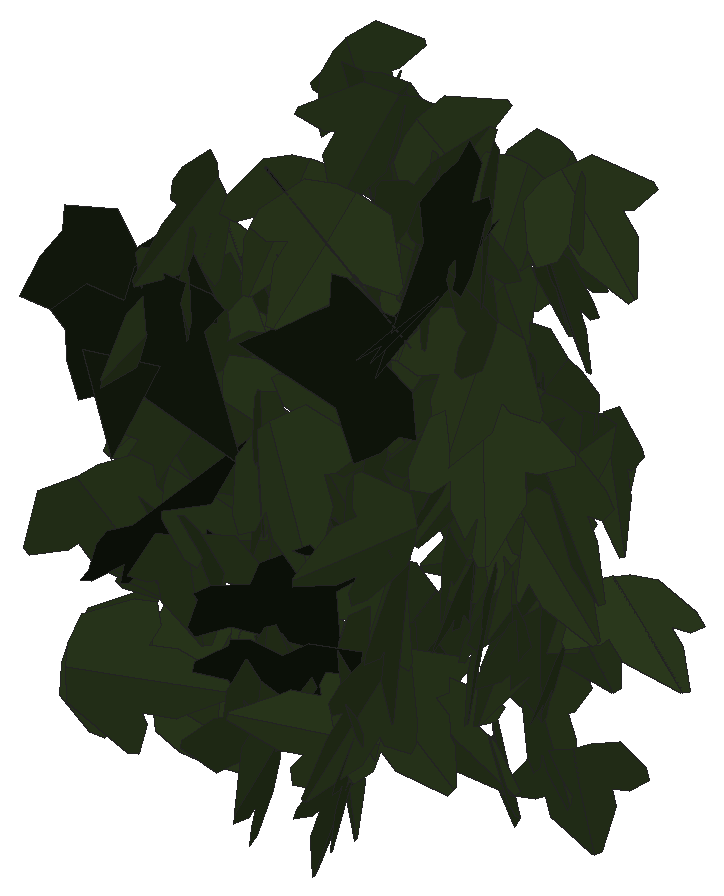
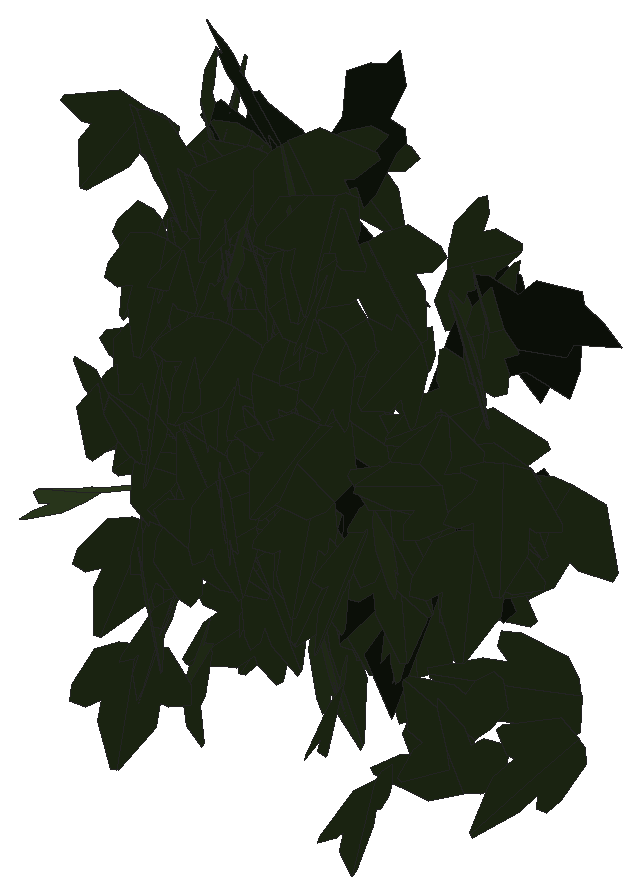
# SketchUp Ruby script. Lengths in inches.
U = 1.inch
M = Sketchup.active_model
def pt(a) = Geom::Point3d.new(a.map { |v| v * U })
def face(e, loops, mat)
  f = e.add_face(loops[0].map { |a| pt(a) })
  loops[1..].each { |l| e.add_face(l.map { |a| pt(a) }).erase! }
  f.material = f.back_material = mat if mat
  f
end
# faces: each face lists its corners as indices into pts; further lists are holes
def faces(e, pts, list, mat = nil) = list.each { |f| face(e, (f[0].is_a?(Array) ? f : [f]).map { |l| l.map { |i| pts[i] } }, mat) }
# xy, xz, yz: faces in a plane at the given z, y or x. An outline is a flat list of corners, or four numbers for a rectangle; further outlines are holes
def ring(l) = l.size == 4 ? [[l[0], l[1]], [l[2], l[1]], [l[2], l[3]], [l[0], l[3]]] : l.each_slice(2).to_a
def flat(e, list, mat, &to3) = list.each { |f| face(e, (f[0].is_a?(Array) ? f : [f]).map { |l| ring(l).map { |u, v| to3.(u, v) } }, mat) }
def xy(e, z, list, mat = nil) = flat(e, list, mat) { |x, y| [x, y, z] }
def xz(e, y, list, mat = nil) = flat(e, list, mat) { |x, z| [x, y, z] }
def yz(e, x, list, mat = nil) = flat(e, list, mat) { |y, z| [x, y, z] }
def lines(e, pts, list) = list.each { |a, b| e.add_line(pt(pts[a]), pt(pts[b])) }
# prism: a flat outline (further loops are holes) pulled along v
def prism(e, loops, v, mat = nil)
  f = face(e, loops, mat); d = Geom::Vector3d.new(v.map { |x| x * U })
  f.pushpull(f.normal.samedirection?(d) ? d.length : -d.length)
end
def box(e, o, s, mat = nil) = prism(e, [[o, [o[0] + s[0], o[1], o[2]], [o[0] + s[0], o[1] + s[1], o[2]], [o[0], o[1] + s[1], o[2]]]], [0, 0, s[2]], mat)
def at(x, y, z, deg = 0) = Geom::Transformation.translation(pt([x, y, z])) * Geom::Transformation.rotation(ORIGIN, Z_AXIS, deg.degrees)
def axes(o, x, y, z) = Geom::Transformation.new([*x, 0, *y, 0, *z, 0, *pt(o).to_a, 1])
def part(name) = M.definitions.add(name)
# library, detail: a bought-in or finely detailed component or shape, given as its bounding box
def library(name, o, s) = part(name).tap { |d| box(d.entities, o, s) }
def detail(e, o, s) = box(e.add_group.entities, o, s)
def put(e, d, t, mat = nil) = e.add_instance(d, t).tap { |i| i.material = mat if mat }
def group(e, t, mat = nil) = e.add_group.tap { |g| g.transformation = t; g.material = mat if mat }.entities
root = M.entities
M.materials.add("efeu1").color = [18, 25, 13]
M.materials.add("efeu2").color = [43, 57, 29]
c1 = part("ivyleaf_10")
p = [[0,0.5,-0.03],[-0.0625,2.02,-0.43],[-0.19,2.01,-0.46],[-0.54,1.05,-0.29],[-0.52,0.625,-0.18],[-0.83,0.76,-0.28],
  [-1.16,0.64,-0.33],[-1.15,0.33,-0.24],[-0.77,-0.39,0.02],[-0.3,-0.51,0.16],[0.04,-0.48,0.23],[-0.02,2.01,-0.4375],
  [-0.06,2.01,-0.43],[0.04,-0.49,0.23],[0.67,-0.49,0.14],[1.38,0.36,-0.2],[1.375,0.51,-0.24],[0.81,0.65,-0.19],
  [0.62,0.59,-0.15],[0.6,1.09,-0.28],[0.5,1.23,-0.31]]
faces(c1.entities,p,[[0,1,2,3,4,5,6,7,8,9,10],[11,12,0,13,14,15,16,17,18,19,20]],"efeu2")
c2 = part("ivyleaf_9")
p = [[1.54,2.16,1.25],[1.36,2.04,1.19],[-0.21,0.99,0.68],[-0.71,1.11,0.82],[-0.85,0.86,0.67],[-0.8,0.17,0.21],
  [-0.9,-0.01,0.1],[-0.67,-0.16,-0.02],[-0.08,-0.08,-0.05],[-0.03,-0.6,-0.4],[0.65,-0.88,-0.66],[0.83,-0.6,-0.49],
  [1.29,-0.42,-0.43],[1.8125,-0.07,-0.26],[1.21,0.44,0.15]]
faces(c2.entities,p,[[0,1,2,3,4,5,6,7,8,9,10,11,12,13,14]],"efeu1")
put(root,c1,axes([598.12,137.04,169.68],[-0.00094,-0.16747,0.7103],[0.19279,-0.68513,-0.16128],[0.70385,0.18744,0.04512]))
put(root,c2,axes([597.98,136.37,169.84],[-0.18069,-0.20058,-0.71209],[0.44721,0.55432,-0.26962],[0.58933,-0.48214,-0.01373]))
put(root,c2,axes([597.75,136.77,170.26],[-0.54152,-0.45185,-0.36971],[0.27813,0.24371,-0.70523],[0.51332,-0.60872,-0.00792]))
put(root,c1,axes([599.44,137.05,164.22],[-0.10246,0.01438,0.77216],[0.4757,-0.61244,0.07452],[0.60839,0.48129,0.07177]))
put(root,c1,axes([599.68,136.74,168.8],[-0.16104,0.54448,-0.30768],[0.07215,-0.29943,-0.56763],[-0.62123,-0.17592,0.01384]))
put(root,c1,axes([598.22,137.02,169.99],[0.02528,-0.04858,-0.68437],[0.3438,-0.59175,0.05471],[-0.59374,-0.34472,0.00254]))
put(root,c2,axes([600.16,136.57,171.97],[0.70624,-0.29216,-0.01882],[-0.01644,0.00948,-0.76428],[0.2923,0.70642,0.00247]))
put(root,c2,axes([601.4,136.67,170.17],[-0.23014,0.01953,-0.72477],[-0.64627,-0.35021,0.19577],[-0.32865,0.67499,0.12254]))
put(root,c1,axes([597.39,136.52,167.09],[-0.59466,-0.39368,-0.37778],[0.34415,0.16298,-0.71156],[0.42339,-0.6854,0.04779]))
put(root,c1,axes([600.03,136.57,168.53],[0.16273,0.7537,0.11512],[0.02463,0.11246,-0.77107],[-0.76204,0.16458,-0.00034]))
put(root,c1,axes([599.46,136.9,164.56],[-0.29472,-0.72736,-0.06906],[-0.02636,-0.06383,0.7848],[-0.73015,0.2959,-0.00046]))
put(root,c1,axes([600.63,137.0625,164.85],[0.08816,0.13501,0.65877],[-0.4395,-0.49131,0.1595],[0.50897,-0.44763,0.02363]))
put(root,c1,axes([601.49,136.92,167.0625],[0.31671,-0.70982,0.08083],[0.16055,-0.01543,-0.76463],[0.69613,0.3265,0.13958]))
put(root,c2,axes([597.81,136.625,166.375],[0.31189,0.68993,0.05468],[-0.04652,-0.03895,0.75669],[0.69052,-0.31425,0.02628]))
put(root,c1,axes([601.01,137.19,165.58],[0.02451,0.54049,-0.53466],[-0.26029,-0.49664,-0.51399],[-0.71431,0.19953,0.16895]))
put(root,c1,axes([600.49,137.04,171.55],[0.60036,0.27951,-0.31616],[-0.28387,-0.13931,-0.66221],[-0.31225,0.66407,-0.00585]))
put(root,c2,axes([602.32,137.12,172.32],[-0.67019,0.21596,-0.35153],[0.32806,-0.12767,-0.70388],[-0.25017,-0.74594,0.0187]))
put(root,c1,axes([600.92,137.42,167.41],[-0.02445,-0.02156,0.66723],[-0.01179,-0.66756,-0.022],[0.66747,-0.01258,0.02405]))
put(root,c1,axes([598.27,137.41,170.9],[0.0302,0.25247,-0.67775],[-0.11166,-0.66857,-0.25403],[-0.71457,0.11515,0.01106]))
put(root,c2,axes([600,136.68,165.81],[0.37753,0.58895,-0.35695],[-0.29716,-0.22791,-0.69033],[-0.62127,0.4669,0.11329]))
put(root,c1,axes([598.33,137.03,167.96],[-0.56505,-0.28517,0.36611],[-0.32868,-0.16131,-0.63292],[0.32761,-0.65368,-0.00353]))
put(root,c2,axes([602.11,136.92,171.36],[-0.46704,0.62886,-0.13687],[-0.02331,-0.18552,-0.77289],[-0.64316,-0.44993,0.12739]))
put(root,c2,axes([599.72,136.51,166.75],[0.45051,0.6646,0.04239],[0.02729,0.03271,-0.80289],[-0.66539,0.45132,-0.00423]))
put(root,c1,axes([598.26,137.07,166.2],[-0.51043,0.08714,-0.52601],[-0.52695,0.02846,0.51607],[0.08121,0.7324,0.04253]))
put(root,c1,axes([597.2,136.88,164.63],[-0.03493,-0.00707,-0.79493],[0.78918,0.09553,-0.03553],[0.09575,-0.78994,0.00281]))
put(root,c1,axes([598.38,137.01,166.47],[-0.57362,-0.34446,-0.03193],[0.02728,0.01659,-0.6691],[0.34486,-0.57427,-0.00018]))
put(root,c1,axes([602.31,137.39,170.84],[-0.33697,0.46787,0.50899],[0.30301,-0.409,0.57656],[0.62141,0.45314,-0.00513]))
put(root,c1,axes([600.5,137.27,164.4],[0.17307,-0.73707,0.09646],[-0.00535,-0.10027,-0.75661],[0.74334,0.17089,-0.02791]))
put(root,c1,axes([600.52,137.39,164.75],[0.39169,-0.63117,0.09926],[0.06472,-0.07664,-0.74269],[0.63564,0.39673,0.01446]))
put(root,c1,axes([601.74,137.69,167.62],[-0.04421,-0.28985,-0.63625],[0.32943,-0.57095,0.23721],[-0.61669,-0.28422,0.17233]))
put(root,c1,axes([599.38,137.31,165.3125],[-0.45285,0.32436,-0.36513],[0.30643,-0.19903,-0.55685],[-0.3803,-0.54661,-0.01391]))
put(root,c1,axes([600.68,137.07,165.8],[-0.26645,0.49635,0.38567],[-0.22343,0.31674,-0.562],[-0.58752,-0.34556,0.03883]))
put(root,c1,axes([602.18,137.51,170.26],[0.74901,0.04342,-0.11895],[-0.11994,0.01445,-0.74997],[-0.04061,0.75826,0.02111]))
put(root,c1,axes([598.02,137.64,170.22],[0.47169,-0.57647,-0.03784],[-0.02352,0.02965,-0.74486],[0.57723,0.47228,0.00057]))
put(root,c1,axes([598.53,137.59,168.26],[-0.19879,-0.0151,-0.63074],[0.61622,-0.14657,-0.1907],[-0.1354,-0.64488,0.05811]))
put(root,c1,axes([598.34,137.11,167.36],[-0.00658,0.49727,0.53231],[-0.02821,0.53176,-0.4971],[-0.7279,-0.0251,0.01446]))
put(root,c1,axes([602.18,137.5625,169.11],[0.53495,0.52861,0.02722],[0.01948,0.01902,-0.75206],[-0.52895,0.5353,-0.00016]))
put(root,c1,axes([601.92,137.9375,166.67],[0.36629,-0.32575,0.49459],[0.34918,-0.35092,-0.48973],[0.47834,0.50562,-0.02125]))
put(root,c1,axes([597.71,137.64,168.11],[0.55127,-0.0916,-0.40363],[-0.40034,0.05261,-0.55871],[0.10504,0.68121,-0.01112]))
put(root,c1,axes([600.5,137.71,166.33],[0.68399,-0.2207,-0.05303],[-0.04822,0.02324,-0.71868],[0.2218,0.68565,0.00729]))
put(root,c1,axes([599.8,137.98,168.31],[-0.23048,-0.28788,0.54307],[-0.32592,-0.4345,-0.36865],[0.52113,-0.39907,0.00963]))
put(root,c1,axes([598.37,137.21,168.58],[0.02744,-0.07316,0.66296],[-0.05757,0.66079,0.0753],[-0.6645,-0.06027,0.02086]))
put(root,c1,axes([601.9,138.05,172.12],[0.34235,-0.40903,0.4743],[0.37577,-0.29829,-0.52848],[0.50106,0.50317,0.07227]))
put(root,c1,axes([600.875,137.38,165.3],[0.28122,0.56152,0.42564],[0.10198,0.42103,-0.62281],[-0.69719,0.28808,0.08059]))
put(root,c1,axes([601.64,137.75,171.46],[-0.67701,0.08676,-0.08449],[0.08282,-0.01835,-0.6825],[-0.08835,-0.68201,0.00762]))
put(root,c1,axes([601.78,137.82,167.12],[0.16628,-0.57663,-0.35816],[-0.10484,0.3425,-0.60011],[0.67066,0.19651,-0.00501]))
put(root,c1,axes([601.08,137.99,166.36],[-0.50462,-0.05558,0.38763],[-0.38182,-0.07059,-0.50717],[0.08698,-0.63239,0.02255]))
put(root,c1,axes([601.42,137.63,171.13],[0.19483,-0.42232,-0.55143],[0.02762,0.57697,-0.43212],[0.69402,0.0956,0.172]))
put(root,c1,axes([600.51,137.72,167.77],[-0.33742,0.41011,0.36563],[-0.22972,0.28446,-0.53107],[-0.49911,-0.40818,-0.00275]))
put(root,c1,axes([600.75,138.24,165.62],[-0.0006,-0.65883,0.16871],[0.00446,-0.16871,-0.65881],[0.68007,0.00052,0.00447]))
put(root,c1,axes([599.04,138.13,170.99],[0.4283,0.49079,-0.25962],[-0.26584,-0.10659,-0.64007],[-0.48745,0.48937,0.12095]))
put(root,c1,axes([599.74,138.12,164.24],[-0.18973,0.57199,-0.22008],[0.08381,-0.20401,-0.60246],[-0.60711,-0.20692,-0.01439]))
put(root,c1,axes([598.625,138.09,169.68],[-0.49263,0.25831,-0.34202],[0.30586,-0.15315,-0.55622],[-0.30025,-0.57983,-0.00546]))
put(root,c1,axes([596.53,137.59,164.24],[0.07282,0.38468,0.60598],[0.09011,0.59937,-0.39131],[-0.71209,0.11518,0.01245]))
put(root,c1,axes([601.12,138.03,164.91],[-0.44738,-0.05685,-0.4497],[0.45027,0.01689,-0.45009],[0.0521,-0.63411,0.02833]))
put(root,c1,axes([597.9,137.94,163.63],[0.63713,0.3037,-0.20744],[0.18744,0.08888,0.70581],[0.31644,-0.66413,-0.00041]))
put(root,c1,axes([601.05,138.375,168.23],[-0.03152,-0.60197,0.25097],[-0.016,-0.25048,-0.60279],[0.652,-0.03524,-0.00266]))
put(root,c1,axes([597.26,138.45,167.41],[0.04502,0.48939,-0.48758],[-0.24893,-0.4443,-0.46893],[-0.64441,0.20582,0.14708]))
put(root,c1,axes([598.59,138.48,167.34],[0.24763,-0.54842,0.35009],[0.16405,-0.30985,-0.60144],[0.62961,0.29643,0.01901]))
put(root,c1,axes([598.75,138.14,166.65],[-0.63625,-0.16491,0.17004],[-0.16403,-0.04484,-0.65727],[0.17089,-0.65705,0.00218]))
put(root,c1,axes([602.01,138.29,168.97],[-0.02467,-0.66145,0.00259],[-0.00035,-0.00258,-0.66191],[0.66145,-0.02468,-0.00026]))
put(root,c1,axes([601.89,138.37,169.15],[-0.55591,0.03531,0.40065],[0.39258,-0.10097,0.55362],[0.08745,0.67777,0.0616]))
put(root,c1,axes([600.66,138.41,171.51],[0.52729,-0.43545,0.13857],[0.09796,-0.09895,-0.68371],[0.44634,0.53614,-0.01364]))
put(root,c1,axes([597.84,137.82,164.27],[0.26991,0.4724,-0.5018],[0.24465,0.43814,0.54406],[0.64429,-0.36427,0.00363]))
put(root,c1,axes([601.36,138.47,170.94],[0.41173,-0.49402,0.15947],[0.11382,-0.11267,-0.64293],[0.50649,0.42691,0.01485]))
put(root,c1,axes([601.37,138.27,169.07],[-0.40626,-0.55467,-0.06132],[0.04241,0.04495,-0.68749],[0.55643,-0.40839,0.00762]))
put(root,c1,axes([601.98,138.22,166.56],[-0.23956,0.05717,0.6395],[-0.64186,-0.00475,-0.24002],[-0.0156,-0.68288,0.05521]))
put(root,c1,axes([600.05,138.49,172.16],[-0.39575,-0.51057,0.28851],[-0.16148,-0.23974,-0.64575],[0.56378,-0.42707,0.01757]))
put(root,c1,axes([602.08,138.48,166.42],[0.1352,0.61816,-0.31897],[-0.21167,-0.27297,-0.61873],[-0.66261,0.21333,0.13257]))
put(root,c1,axes([602.57,138.4375,168.24],[-0.55836,0.16877,-0.41205],[0.33894,-0.2675,-0.56886],[-0.28877,-0.64031,0.12904]))
put(root,c1,axes([600.77,138.19,171.13],[-0.19534,-0.54751,0.36877],[0.11106,0.35184,0.5812],[-0.65071,0.22441,-0.01151]))
put(root,c1,axes([602.2,138.83,167.07],[-0.03471,-0.32985,0.54581],[0.10527,-0.54208,-0.3209],[0.62899,0.07253,0.08383]))
put(root,c1,axes([602.23,138.33,167.51],[0.49285,0.10314,0.51001],[0.48724,0.15507,-0.5022],[-0.18263,0.69207,0.03652]))
put(root,c1,axes([598.84,138.33,167.21],[-0.41155,-0.0235,0.53432],[-0.53363,-0.02726,-0.41222],[0.03594,-0.67389,-0.00195]))
put(root,c1,axes([600.78,138.59,170.97],[0.4377,-0.51157,0.11609],[0.06548,-0.09673,-0.67314],[0.52047,0.44238,-0.01294]))
put(root,c1,axes([596.79,138.42,168.45],[-0.68938,-0.1225,0.08321],[-0.07423,-0.05701,-0.69887],[0.12815,-0.69204,0.04284]))
put(root,c1,axes([599.62,138.47,166.33],[-0.5707,0.2669,-0.16946],[0.14943,-0.08047,-0.62996],[-0.27862,-0.58987,0.00926]))
put(root,c1,axes([600.4,138.61,170.5],[0.6737,0.02357,-0.00614],[-0.00534,-0.02288,-0.67373],[-0.02377,0.67334,-0.02268]))
put(root,c1,axes([602.18,138.57,166.17],[-0.06177,-0.69089,-0.10099],[0.07403,0.09433,-0.69063],[0.6943,-0.07153,0.06465]))
put(root,c1,axes([601.76,138.68,171.67],[0.66153,-0.13423,-0.04557],[-0.04407,0.01198,-0.67501],[0.13473,0.66299,0.00297]))
put(root,c1,axes([601.93,138.78,168.83],[-0.4816,-0.29861,0.35694],[-0.25111,-0.26572,-0.56111],[0.39181,-0.53734,0.07912]))
put(root,c1,axes([601.28,138.6,171.23],[0.36232,-0.51699,-0.24102],[-0.082,0.23535,-0.62812],[0.56449,0.36603,0.06345]))
put(root,c1,axes([597.03,138.67,167.48],[-0.49051,-0.48389,-0.056],[0.05089,0.02813,-0.68884],[0.48445,-0.4929,0.01566]))
put(root,c1,axes([600.32,138.6,171.04],[-0.52729,0.41618,0.11689],[-0.13655,0.01458,-0.66787],[-0.41015,-0.5399,0.07207]))
put(root,c1,axes([602.3,138.76,172.03],[0.61996,-0.2508,-0.17565],[-0.15214,0.09191,-0.66822],[0.26572,0.63778,0.02722]))
put(root,c1,axes([600.87,138.83,170.52],[-0.37299,0.49609,0.18125],[0.10295,-0.14935,0.62062],[0.51803,0.38687,0.00717]))
put(root,c1,axes([602.71,138.58,171.96],[0.44865,0.33923,0.36591],[0.29062,0.22233,-0.56245],[-0.40559,0.53455,0.00173]))
put(root,c1,axes([599.45,138.32,169.86],[0.24064,0.15755,0.56905],[0.1932,0.55966,-0.23664],[-0.55795,0.26174,0.16348]))
put(root,c1,axes([599.46,138.82,168.22],[0.21021,-0.04963,-0.60136],[0.57734,-0.1686,0.21573],[-0.17543,-0.61433,-0.01062]))
put(root,c1,axes([599.58,138.97,171.34],[0.34079,-0.44059,-0.36727],[0.23021,-0.28622,0.55698],[-0.52537,-0.41122,0.00583]))
put(root,c1,axes([599.29,138.78,169.67],[-0.58233,0.29558,-0.19809],[0.1754,-0.0921,-0.65304],[-0.30959,-0.60816,0.00262]))
put(root,c1,axes([601.75,138.57,163.89],[-0.30209,0.38808,-0.44475],[-0.25734,0.36304,0.49158],[0.53121,0.39656,-0.01478]))
put(root,c1,axes([603.01,139.17,166.51],[-0.27683,-0.62901,0.01414],[0.62005,-0.27537,-0.11044],[0.10673,-0.03172,0.6783]))
put(root,c1,axes([600.85,139.27,167.68],[-0.1439,-0.45275,0.43683],[-0.05655,-0.43699,-0.47154],[0.62658,-0.14341,0.05777]))
put(root,c1,axes([600.62,138.66,171.92],[0.16877,0.51805,0.38799],[0.06891,0.3843,-0.5431],[-0.64356,0.17701,0.0436]))
put(root,c1,axes([599.81,139.43,169.5],[0.07955,-0.33999,0.5387],[0.21978,-0.4949,-0.3448],[0.5979,0.22716,0.05507]))
put(root,c1,axes([599.68,138.78,167.18],[0.0641,0.61309,0.20589],[-0.16189,0.21552,-0.59138],[-0.62615,0.00704,0.17398]))
put(root,c1,axes([602.01,138.9,164.97],[-0.14443,0.63364,0.06608],[-0.01206,0.06502,-0.64989],[-0.63696,-0.14491,-0.00268]))
put(root,c1,axes([597.41,138.61,168.42],[-0.00829,-0.19145,0.674],[0.14405,0.65918,0.18901],[-0.68569,0.14079,0.03156]))
put(root,c1,axes([602.14,139.03,165.66],[0.26112,-0.55773,-0.19964],[-0.08666,0.17987,-0.61582],[0.58601,0.27511,-0.00211]))
put(root,c1,axes([600.86,139.07,169.1875],[-0.12149,-0.6408,-0.11356],[0.07302,0.10137,-0.65013],[0.64667,-0.13183,0.05208]))
put(root,c1,axes([597.76,139.08,168.35],[0.40984,0.50459,0.164],[-0.10323,-0.12743,0.65006],[0.52043,-0.42265,-0.0002]))
put(root,c1,axes([600.49,138.99,168.85],[-0.24433,0.58998,0.13728],[-0.28621,0.01802,-0.58684],[-0.53386,-0.27968,0.25178]))
put(root,c1,axes([602.09,139.0625,170.63],[-0.54001,0.33285,-0.11259],[0.09109,-0.06676,-0.63429],[-0.33936,-0.54757,0.0089]))
put(root,c1,axes([600.67,139.2,167.85],[-0.3776,-0.51329,0.03968],[0.02631,-0.06838,-0.63424],[0.51415,-0.37347,0.06159]))
put(root,c1,axes([601.27,138.93,170.6],[0.01875,0.63747,0.18583],[-0.04041,0.18665,-0.63622],[-0.66277,0.00666,0.04405]))
put(root,c1,axes([602.33,139.125,164.16],[-0.50048,-0.42141,-0.07898],[0.0595,0.05195,-0.65427],[0.4246,-0.504,-0.00141]))
put(root,c1,axes([598.89,138.88,166.97],[-0.18971,0.57444,0.29303],[-0.09943,0.27574,-0.60492],[-0.63716,-0.21406,0.00715]))
put(root,c1,axes([602.4,139.34,168.3],[0.24139,0.35743,-0.47239],[-0.47309,-0.19067,-0.38601],[-0.3565,0.49504,0.1924]))
put(root,c1,axes([601.3125,139.32,166.52],[-0.20894,-0.06185,0.6089],[-0.54987,-0.26354,-0.21545],[0.26874,-0.58733,0.03256]))
put(root,c1,axes([599.22,139.15,168.07],[-0.36543,-0.21605,0.5068],[0.46294,0.20928,0.42302],[-0.29868,0.58871,0.03561]))
put(root,c1,axes([602.01,139.24,169.16],[-0.51149,0.0438,0.39046],[-0.3929,-0.06202,-0.50773],[0.00307,-0.6405,0.07586]))
put(root,c1,axes([599.27,139.2,171.89],[-0.66135,-0.06659,-0.00009],[0.00009,0.00003,-0.6647],[0.06659,-0.66135,-0.00002]))
put(root,c1,axes([602.16,139.22,166.11],[-0.46066,-0.39192,-0.22314],[0.18711,0.12414,-0.6043],[0.41034,-0.49658,0.02505]))
put(root,c1,axes([601.71,139.22,168.66],[0.19417,-0.58124,-0.23123],[0.09575,0.26688,-0.59044],[0.61817,0.14123,0.16409]))
put(root,c1,axes([602.38,139.52,168.24],[0.51182,-0.10442,0.37587],[0.36767,-0.07812,-0.52236],[0.13039,0.63018,-0.00247]))
put(root,c1,axes([600.51,139.45,167.57],[0.42203,-0.49123,0.03566],[0.11839,0.0556,-0.63528],[0.47808,0.41987,0.12584]))
put(root,c1,axes([599.41,139.15,168.61],[0.27523,0.48236,0.34661],[0.15652,0.30962,-0.55516],[-0.57298,0.31628,0.01484]))
put(root,c1,axes([600.47,139.54,167.42],[-0.1329,-0.62239,0.09259],[0.01399,-0.09753,-0.63553],[0.62908,-0.12931,0.0337]))
put(root,c1,axes([599.61,139.3125,170.74],[-0.41571,0.18699,-0.46288],[-0.41737,0.2003,0.45576],[0.2739,0.58903,-0.00804]))
put(root,c1,axes([599.03,139.4,171.05],[-0.30207,0.56658,-0.10533],[0.04388,-0.09597,-0.64204],[-0.57461,-0.30517,0.00635]))
put(root,c1,axes([600.625,139.42,169.68],[-0.54487,-0.22754,-0.27438],[0.29063,0.0066,-0.58261],[0.20638,-0.61002,0.09604]))
put(root,c1,axes([598.99,139.24,172.11],[0.12188,0.62067,0.20119],[-0.10692,0.2209,-0.61671],[-0.64364,0.08083,0.14054]))
put(root,c1,axes([600.55,139.54,167.24],[-0.28067,-0.55376,0.16901],[0.08229,0.14777,0.6208],[-0.5731,0.29241,0.00636]))
put(root,c1,axes([601.64,139.47,170.61],[-0.64016,0.0879,0.00655],[-0.00648,0.00098,-0.64617],[-0.0879,-0.6402,-0.00009]))
put(root,c1,axes([598.02,139.6,164],[-0.02632,0.64084,-0.00687],[0.00393,-0.00671,-0.64137],[-0.64087,-0.02636,-0.00365]))
